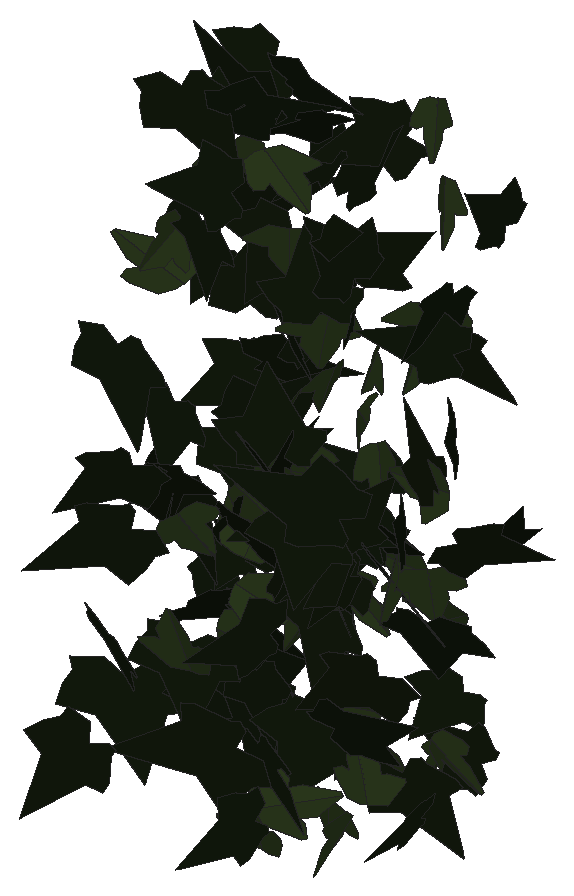
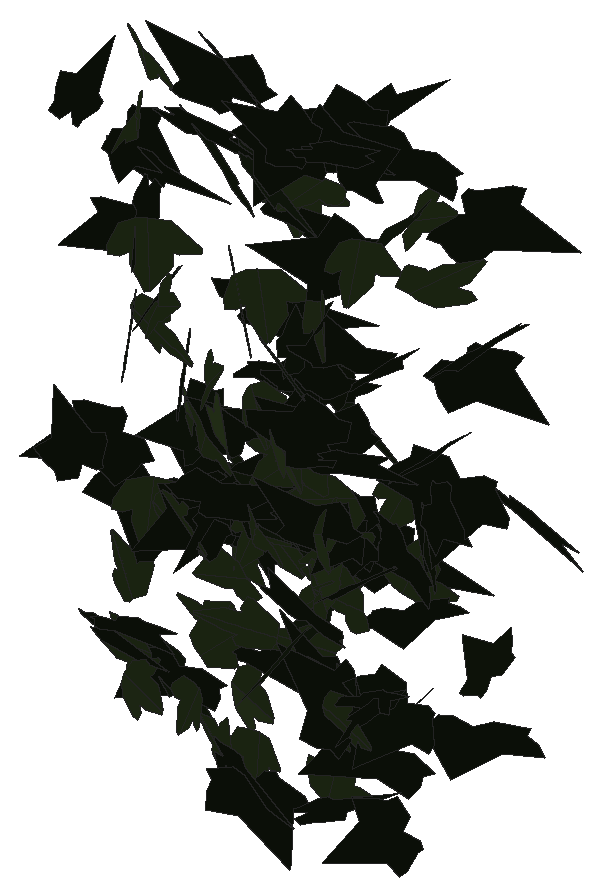
# SketchUp Ruby script. Lengths in inches.
U = 1.inch
M = Sketchup.active_model
def pt(a) = Geom::Point3d.new(a.map { |v| v * U })
def face(e, loops, mat)
  f = e.add_face(loops[0].map { |a| pt(a) })
  loops[1..].each { |l| e.add_face(l.map { |a| pt(a) }).erase! }
  f.material = f.back_material = mat if mat
  f
end
# faces: each face lists its corners as indices into pts; further lists are holes
def faces(e, pts, list, mat = nil) = list.each { |f| face(e, (f[0].is_a?(Array) ? f : [f]).map { |l| l.map { |i| pts[i] } }, mat) }
# xy, xz, yz: faces in a plane at the given z, y or x. An outline is a flat list of corners, or four numbers for a rectangle; further outlines are holes
def ring(l) = l.size == 4 ? [[l[0], l[1]], [l[2], l[1]], [l[2], l[3]], [l[0], l[3]]] : l.each_slice(2).to_a
def flat(e, list, mat, &to3) = list.each { |f| face(e, (f[0].is_a?(Array) ? f : [f]).map { |l| ring(l).map { |u, v| to3.(u, v) } }, mat) }
def xy(e, z, list, mat = nil) = flat(e, list, mat) { |x, y| [x, y, z] }
def xz(e, y, list, mat = nil) = flat(e, list, mat) { |x, z| [x, y, z] }
def yz(e, x, list, mat = nil) = flat(e, list, mat) { |y, z| [x, y, z] }
def lines(e, pts, list) = list.each { |a, b| e.add_line(pt(pts[a]), pt(pts[b])) }
# prism: a flat outline (further loops are holes) pulled along v
def prism(e, loops, v, mat = nil)
  f = face(e, loops, mat); d = Geom::Vector3d.new(v.map { |x| x * U })
  f.pushpull(f.normal.samedirection?(d) ? d.length : -d.length)
end
def box(e, o, s, mat = nil) = prism(e, [[o, [o[0] + s[0], o[1], o[2]], [o[0] + s[0], o[1] + s[1], o[2]], [o[0], o[1] + s[1], o[2]]]], [0, 0, s[2]], mat)
def at(x, y, z, deg = 0) = Geom::Transformation.translation(pt([x, y, z])) * Geom::Transformation.rotation(ORIGIN, Z_AXIS, deg.degrees)
def axes(o, x, y, z) = Geom::Transformation.new([*x, 0, *y, 0, *z, 0, *pt(o).to_a, 1])
def part(name) = M.definitions.add(name)
# library, detail: a bought-in or finely detailed component or shape, given as its bounding box
def library(name, o, s) = part(name).tap { |d| box(d.entities, o, s) }
def detail(e, o, s) = box(e.add_group.entities, o, s)
def put(e, d, t, mat = nil) = e.add_instance(d, t).tap { |i| i.material = mat if mat }
def group(e, t, mat = nil) = e.add_group.tap { |g| g.transformation = t; g.material = mat if mat }.entities
root = M.entities
M.materials.add("1026 AP 7946 SUNNY SIDE UP").color = [254, 231, 186]
M.materials.add("efeu1").color = [18, 25, 13]
M.materials.add("efeu2").color = [43, 57, 29]
c1 = part("ivyleaf_9")
p = [[1.54,2.16,1.25],[1.36,2.04,1.19],[-0.21,0.99,0.68],[-0.71,1.11,0.82],[-0.85,0.86,0.67],[-0.8,0.17,0.21],
  [-0.9,-0.01,0.1],[-0.67,-0.16,-0.02],[-0.08,-0.08,-0.05],[-0.03,-0.6,-0.4],[0.65,-0.88,-0.66],[0.83,-0.6,-0.49],
  [1.29,-0.42,-0.43],[1.8125,-0.07,-0.26],[1.21,0.44,0.15]]
faces(c1.entities,p,[[0,1,2,3,4,5,6,7,8,9,10,11,12,13,14]],"efeu1")
c2 = part("ivyleaf_10")
p = [[0,0.5,-0.03],[-0.0625,2.02,-0.43],[-0.19,2.01,-0.46],[-0.54,1.05,-0.29],[-0.52,0.625,-0.18],[-0.83,0.76,-0.28],
  [-1.16,0.64,-0.33],[-1.15,0.33,-0.24],[-0.77,-0.39,0.02],[-0.3,-0.51,0.16],[0.04,-0.48,0.23],[-0.02,2.01,-0.4375],
  [-0.06,2.01,-0.43],[0.04,-0.49,0.23],[0.67,-0.49,0.14],[1.38,0.36,-0.2],[1.375,0.51,-0.24],[0.81,0.65,-0.19],
  [0.62,0.59,-0.15],[0.6,1.09,-0.28],[0.5,1.23,-0.31]]
faces(c2.entities,p,[[0,1,2,3,4,5,6,7,8,9,10],[11,12,0,13,14,15,16,17,18,19,20]],"efeu2")
put(root,c1,axes([141.33,204.3125,274.67],[-0.08778,-0.02071,-0.48621],[-0.04144,-0.47425,0.02188],[-0.74149,0.02896,0.05633]),"1026 AP 7946 SUNNY SIDE UP")
put(root,c1,axes([140.3,204.62,270.57],[-0.70201,0.01951,-0.15809],[0.23469,-0.07018,-0.4566],[-0.0646,-0.46689,0.05923]),"1026 AP 7946 SUNNY SIDE UP")
put(root,c1,axes([142.83,205.35,269.84],[-0.60155,0.20655,-0.09318],[0.095,-0.08009,-0.44638],[-0.34235,-0.38515,0.03986]),"1026 AP 7946 SUNNY SIDE UP")
put(root,c1,axes([141.66,206.34,270.23],[-0.1412,-0.10196,-0.47524],[-0.44551,-0.3634,0.13761],[-0.59335,0.29712,0.00977]),"1026 AP 7946 SUNNY SIDE UP")
put(root,c1,axes([142.4375,206.1875,272.47],[-0.54529,0.329,0.00208],[-0.03997,-0.02658,-0.49115],[-0.51578,-0.34577,0.03587]),"1026 AP 7946 SUNNY SIDE UP")
put(root,c1,axes([139.4375,206.72,273.99],[0.00936,0.11052,-0.39414],[-0.09937,-0.37816,-0.11558],[-0.61921,0.06236,0.01259]),"1026 AP 7946 SUNNY SIDE UP")
put(root,c1,axes([142.97,207.22,270.625],[0.58209,0.0655,-0.17186],[0.22809,0.11671,0.37867],[0.16642,-0.38907,0.08211]),"1026 AP 7946 SUNNY SIDE UP")
put(root,c1,axes([141.375,207.39,269.68],[0.2811,-0.36238,0.03312],[-0.00053,-0.03828,-0.41613],[0.57235,0.17794,-0.01666]),"1026 AP 7946 SUNNY SIDE UP")
put(root,c1,axes([142.76,207.38,274.05],[-0.27783,0.07056,0.43166],[-0.65081,0.07215,-0.19208],[-0.14837,-0.44861,0.03424]),"1026 AP 7946 SUNNY SIDE UP")
put(root,c2,axes([139.95,207.39,270.67],[-0.56819,0.04904,-0.0988],[-0.14095,0.05096,0.37402],[0.0946,0.37045,-0.03612]),"1026 AP 7946 SUNNY SIDE UP")
put(root,c2,axes([141.7,207.24,268.91],[0.23552,-0.00672,-0.37454],[0.52266,0.16187,0.13896],[0.23169,-0.35831,0.06727]),"1026 AP 7946 SUNNY SIDE UP")
put(root,c1,axes([142.05,207.64,273.49],[-0.32105,-0.33925,-0.05283],[0.06514,0.03261,-0.40727],[0.5351,-0.20751,0.01788]),"1026 AP 7946 SUNNY SIDE UP")
put(root,c1,axes([138.36,207.82,275.13],[0.01346,-0.47992,0.01511],[0.01074,-0.01727,-0.49454],[0.75505,0.0088,0.00676]),"1026 AP 7946 SUNNY SIDE UP")
put(root,c1,axes([139.62,207.92,270.54],[-0.23506,-0.40184,-0.07874],[0.04593,0.06824,-0.44128],[0.64088,-0.15228,0.00275]),"1026 AP 7946 SUNNY SIDE UP")
put(root,c1,axes([138.04,207.99,270.125],[0.09553,-0.26086,0.27989],[0.13003,-0.26078,-0.27703],[0.57951,0.10151,0.01602]),"1026 AP 7946 SUNNY SIDE UP")
put(root,c1,axes([143.1,207.92,271.24],[0.09585,0.06198,-0.39943],[-0.34043,-0.32245,-0.08997],[-0.51571,0.22437,-0.01485]),"1026 AP 7946 SUNNY SIDE UP")
put(root,c1,axes([140.16,208.125,278.26],[-0.19778,-0.06121,0.4093],[-0.42491,-0.29581,-0.1367],[0.46869,-0.29401,0.04878]),"1026 AP 7946 SUNNY SIDE UP")
put(root,c2,axes([142.33,208.1,268.39],[0.1333,-0.29257,0.2564],[0.08138,-0.24556,-0.31489],[0.60018,0.09828,-0.01425]),"1026 AP 7946 SUNNY SIDE UP")
put(root,c2,axes([139.09,208.25,277.16],[0.09776,0.14683,-0.37943],[-0.14773,-0.3576,-0.16493],[-0.60695,0.11069,-0.02097]),"1026 AP 7946 SUNNY SIDE UP")
put(root,c2,axes([139.48,207.95,272.59],[-0.26698,-0.28775,-0.20995],[0.21357,0.15342,-0.34158],[0.51006,-0.21486,0.03313]),"1026 AP 7946 SUNNY SIDE UP")
put(root,c1,axes([142.77,207.79,277.94],[-0.13686,0.27393,0.38347],[-0.27002,0.33079,-0.29144],[-0.67255,-0.18855,0.03898]),"1026 AP 7946 SUNNY SIDE UP")
put(root,c1,axes([140.6875,208.06,274.11],[0.54317,-0.17404,-0.10493],[-0.16391,0.01655,-0.3971],[0.27051,0.35949,-0.02992]),"1026 AP 7946 SUNNY SIDE UP")
put(root,c1,axes([142.01,207.98,277.03],[-0.5582,-0.07882,0.12233],[0.16876,0.06367,0.37306],[-0.14835,0.36902,-0.03592]),"1026 AP 7946 SUNNY SIDE UP")
put(root,c1,axes([138.15,208.23,269.32],[-0.34763,-0.35399,-0.24935],[0.23608,0.18878,-0.42816],[0.62972,-0.26619,0.02286]),"1026 AP 7946 SUNNY SIDE UP")
put(root,c2,axes([142.84,208.04,269.21],[0.53812,-0.01345,0.14735],[-0.21966,0.0559,0.3499],[-0.05322,-0.36671,0.04573]),"1026 AP 7946 SUNNY SIDE UP")
put(root,c1,axes([138.57,208.05,273.03],[0.5327,0.28218,-0.10711],[-0.09377,-0.09292,-0.45354],[-0.46437,0.34247,-0.03129]),"1026 AP 7946 SUNNY SIDE UP")
put(root,c1,axes([142.54,208.16,277.88],[-0.15475,0.02402,0.40412],[0.59348,-0.10642,0.10368],[0.17146,0.39004,0.00586]),"1026 AP 7946 SUNNY SIDE UP")
put(root,c2,axes([140.62,208.26,267.5],[-0.53757,0.06449,-0.03595],[-0.04669,0.0323,0.35759],[0.10572,0.34217,-0.02489]),"1026 AP 7946 SUNNY SIDE UP")
put(root,c1,axes([141.7,208.55,271.54],[-0.15537,-0.37938,0.12184],[-0.03131,-0.11921,-0.40443],[0.62508,-0.10027,0.01003]),"1026 AP 7946 SUNNY SIDE UP")
put(root,c2,axes([143.15,208.12,272.3],[0.29387,-0.22552,0.26531],[-0.2243,0.21702,0.3022],[-0.49098,-0.23413,0.02074]),"1026 AP 7946 SUNNY SIDE UP")
put(root,c2,axes([138.74,208.52,276.25],[0.23187,0.26554,0.26408],[-0.25453,-0.19976,0.30976],[0.51973,-0.2163,0.03388]),"1026 AP 7946 SUNNY SIDE UP")
put(root,c1,axes([142.65,208.52,272.73],[0.472,-0.26867,0.0995],[0.07923,-0.09033,-0.41417],[0.44271,0.30261,-0.03197]),"1026 AP 7946 SUNNY SIDE UP")
put(root,c1,axes([141.5625,208.65,269.5],[-0.5956,-0.21258,-0.07549],[0.13602,-0.0078,-0.44472],[0.32568,-0.3855,0.04769]),"1026 AP 7946 SUNNY SIDE UP")
put(root,c1,axes([142.07,208.5625,272.25],[-0.45316,0.13622,-0.19567],[0.22888,-0.13286,-0.32515],[-0.28882,-0.31902,0.04933]),"1026 AP 7946 SUNNY SIDE UP")
put(root,c1,axes([143.46,208.49,268.74],[-0.37016,0.25797,-0.13574],[0.11149,-0.11524,-0.35963],[-0.44271,-0.24472,0.02293]),"1026 AP 7946 SUNNY SIDE UP")
put(root,c1,axes([142.04,208.76,272.22],[-0.21171,-0.21466,0.2554],[-0.18848,-0.21865,-0.2621],[0.48151,-0.17996,0.0097]),"1026 AP 7946 SUNNY SIDE UP")
put(root,c2,axes([141.34,208.68,271.5],[-0.10165,-0.32553,0.18508],[-0.02099,-0.18207,-0.34237],[0.58567,-0.06302,0.01985]),"1026 AP 7946 SUNNY SIDE UP")
put(root,c1,axes([139.12,208.82,277.07],[0.01819,-0.38176,0.18216],[0.00404,-0.17899,-0.39451],[0.66298,0.01156,-0.00259]),"1026 AP 7946 SUNNY SIDE UP")
put(root,c1,axes([141.09,208.3,272.05],[0.00352,0.18396,0.35024],[-0.02228,0.33874,-0.18734],[-0.60597,-0.01139,0.00892]),"1026 AP 7946 SUNNY SIDE UP")
put(root,c1,axes([142.92,208.8,273.07],[-0.03778,0.07812,0.3598],[-0.11961,-0.34271,0.07167],[0.54918,-0.06927,0.04036]),"1026 AP 7946 SUNNY SIDE UP")
put(root,c1,axes([138.8125,208.33,271.96],[-0.00393,0.02888,0.40579],[0.071,0.39118,-0.02698],[-0.6167,0.04485,-0.00569]),"1026 AP 7946 SUNNY SIDE UP")
put(root,c1,axes([138.5,208.92,273.77],[-0.09727,-0.37358,0.14709],[-0.02988,-0.14372,-0.39091],[0.62934,-0.06456,0.00417]),"1026 AP 7946 SUNNY SIDE UP")
put(root,c1,axes([140.78,208.54,273.97],[-0.57491,-0.0912,0.16107],[0.23203,0.0559,0.38813],[-0.16603,0.39391,-0.01531]),"1026 AP 7946 SUNNY SIDE UP")
put(root,c1,axes([138.37,208.82,273.06],[-0.2007,0.12443,-0.32054],[0.31131,-0.24156,-0.18418],[-0.42639,-0.23493,0.0164]),"1026 AP 7946 SUNNY SIDE UP")
put(root,c1,axes([143.86,208.6875,276.61],[-0.39161,0.12928,0.25636],[-0.38266,0.06376,-0.28551],[-0.21702,-0.34572,0.04083]),"1026 AP 7946 SUNNY SIDE UP")
put(root,c1,axes([139.125,209.02,269.19],[0.17762,-0.2802,-0.22578],[0.15576,-0.19434,0.30969],[-0.53563,-0.14943,0.01518]),"1026 AP 7946 SUNNY SIDE UP")
put(root,c2,axes([141.09,208.52,272.3125],[0.15454,0.01027,-0.38752],[-0.32787,0.32519,-0.04507],[0.49267,0.21319,0.09157]),"1026 AP 7946 SUNNY SIDE UP")
put(root,c1,axes([143.5625,208.66,274.3],[-0.15825,-0.27823,0.28306],[0.11036,0.26791,0.30579],[-0.60666,0.12132,-0.01821]),"1026 AP 7946 SUNNY SIDE UP")
put(root,c2,axes([141,208.76,273.41],[-0.58887,0.07318,-0.0741],[0.10129,-0.04621,-0.39196],[-0.12619,-0.37862,0.03119]),"1026 AP 7946 SUNNY SIDE UP")
put(root,c1,axes([139.68,208.85,272.16],[0.57429,-0.16064,0.1972],[0.24833,-0.11639,-0.40979],[0.30593,0.39603,-0.03754]),"1026 AP 7946 SUNNY SIDE UP")
put(root,c1,axes([140.79,208.48,273.54],[0.03377,0.10674,0.43817],[0.26161,0.39136,-0.1077],[-0.63697,0.16639,-0.021]),"1026 AP 7946 SUNNY SIDE UP")
put(root,c1,axes([138.72,209.01,272.29],[-0.2018,-0.05634,-0.41322],[0.63639,-0.02104,-0.13059],[-0.00481,-0.42031,0.05942]),"1026 AP 7946 SUNNY SIDE UP")
put(root,c1,axes([140.05,208.97,269.76],[-0.31353,-0.05901,-0.32266],[0.49225,0.03089,-0.21136],[0.09117,-0.36971,0.0316]),"1026 AP 7946 SUNNY SIDE UP")
put(root,c1,axes([143.61,209.05,277.3],[-0.11365,0.14194,-0.36763],[0.23252,-0.32572,-0.16586],[-0.55858,-0.16446,0.00575]),"1026 AP 7946 SUNNY SIDE UP")
put(root,c2,axes([143.55,208.74,274.22],[0.13498,-0.12002,-0.37317],[-0.44601,0.22726,-0.14577],[0.39986,0.29401,-0.03662]),"1026 AP 7946 SUNNY SIDE UP")
put(root,c2,axes([141.56,208.8125,268.13],[-0.47815,0.14381,0.06997],[-0.11414,0.00293,-0.34533],[-0.22191,-0.31139,0.02686]),"1026 AP 7946 SUNNY SIDE UP")
put(root,c1,axes([141.14,208.5625,271.84],[-0.33674,0.24858,-0.24937],[-0.2091,0.20572,0.33808],[0.50559,0.25064,-0.02627]),"1026 AP 7946 SUNNY SIDE UP")
put(root,c2,axes([140.73,208.89,277.375],[-0.4632,-0.21263,0.00481],[0.0193,-0.02701,-0.37323],[0.33392,-0.2934,0.02824]),"1026 AP 7946 SUNNY SIDE UP")
put(root,c1,axes([141.84,208.72,272.87],[-0.18998,-0.03852,0.35846],[0.49055,0.15567,0.13018],[-0.2505,0.33405,-0.01693]),"1026 AP 7946 SUNNY SIDE UP")
put(root,c2,axes([139.92,208.98,272.7],[-0.32259,0.0313,-0.32034],[0.45626,-0.11964,-0.21021],[-0.18326,-0.35295,0.04053]),"1026 AP 7946 SUNNY SIDE UP")
put(root,c2,axes([140.07,208.76,271.22],[0.13487,0.22376,0.26759],[0.16524,0.23633,-0.24531],[-0.51155,0.13533,-0.00869]),"1026 AP 7946 SUNNY SIDE UP")
put(root,c1,axes([142.8,208.99,269],[-0.16714,-0.17706,-0.3564],[0.39561,0.24065,-0.20572],[0.4639,-0.26902,0.04703]),"1026 AP 7946 SUNNY SIDE UP")
put(root,c2,axes([141.75,208.84,271.16],[-0.297,0.19682,-0.25507],[-0.23578,0.19967,0.28127],[0.43947,0.24014,-0.02148]),"1026 AP 7946 SUNNY SIDE UP")
put(root,c2,axes([142.02,209.23,269.71],[-0.14968,-0.09732,-0.31929],[-0.28128,-0.2532,0.13727],[-0.42539,0.20167,0.02158]),"1026 AP 7946 SUNNY SIDE UP")
put(root,c1,axes([139.97,209.15,269.71],[-0.045,0.07556,0.36657],[0.27315,-0.31027,0.08056],[0.50179,0.17567,-0.01098]),"1026 AP 7946 SUNNY SIDE UP")
put(root,c1,axes([143.26,208.97,271.72],[0.50042,0.20049,-0.19467],[-0.22327,-0.13006,-0.38697],[-0.37267,0.34714,-0.02956]),"1026 AP 7946 SUNNY SIDE UP")
put(root,c1,axes([140.41,209.27,277.18],[-0.58202,-0.14266,-0.10119],[0.16388,-0.00073,-0.40689],[0.21663,-0.38275,0.03594]),"1026 AP 7946 SUNNY SIDE UP")
put(root,c2,axes([139.87,208.97,271.88],[0.33375,0.22988,-0.18811],[0.14832,0.16165,0.32128],[0.43849,-0.22965,0.0345]),"1026 AP 7946 SUNNY SIDE UP")
put(root,c1,axes([141.14,209.27,271.82],[-0.125,-0.02486,-0.34638],[0.52959,-0.01765,-0.08083],[-0.01809,-0.34491,0.02707]),"1026 AP 7946 SUNNY SIDE UP")
put(root,c1,axes([139.66,208.91,272.37],[-0.0797,0.06272,-0.36329],[-0.22573,0.32313,0.08227],[0.51659,0.15087,-0.0201]),"1026 AP 7946 SUNNY SIDE UP")
put(root,c1,axes([138.45,209.25,278.89],[-0.22644,-0.17934,-0.39584],[0.50785,0.21491,-0.22739],[0.42978,-0.34844,0.06014]),"1026 AP 7946 SUNNY SIDE UP")
put(root,c1,axes([138.92,209.22,269.15],[-0.06761,-0.12362,-0.41265],[0.42863,0.29674,-0.12298],[0.49937,-0.27144,0.04968]),"1026 AP 7946 SUNNY SIDE UP")
put(root,c2,axes([141.07,209.3125,275.85],[-0.39123,-0.30557,0.02655],[0.00043,-0.03564,-0.40549],[0.48242,-0.24778,0.02189]),"1026 AP 7946 SUNNY SIDE UP")
put(root,c1,axes([140.52,209.53,272.4],[-0.45244,-0.14052,0.17362],[-0.21126,-0.10855,-0.32865],[0.27401,-0.31573,0.03329]),"1026 AP 7946 SUNNY SIDE UP")
put(root,c2,axes([143.17,209.44,269.37],[-0.16186,0.06557,-0.35466],[0.4073,-0.22802,-0.12573],[-0.37203,-0.27817,0.01666]),"1026 AP 7946 SUNNY SIDE UP")
put(root,c2,axes([139.2,209.45,269.92],[0.05677,-0.05771,-0.39558],[0.49181,-0.22366,0.06367],[-0.36096,-0.31381,0.02453]),"1026 AP 7946 SUNNY SIDE UP")
put(root,c2,axes([141.11,209.23,272.07],[-0.17931,-0.3021,-0.21568],[0.16301,0.182,-0.33038],[0.55288,-0.15164,0.02746]),"1026 AP 7946 SUNNY SIDE UP")
put(root,c2,axes([142.21,209.42,268.93],[-0.35925,0.23643,-0.04575],[0.02233,-0.04973,-0.33809],[-0.37799,-0.22764,0.02351]),"1026 AP 7946 SUNNY SIDE UP")
put(root,c2,axes([140.33,209.43,273.42],[-0.48016,-0.04613,-0.20747],[0.32235,-0.02692,-0.31446],[0.03694,-0.36466,0.04728]),"1026 AP 7946 SUNNY SIDE UP")
put(root,c1,axes([143.84,209.4,269.42],[-0.36193,-0.03513,-0.28423],[-0.43614,0.00628,0.23777],[-0.02778,0.3591,-0.02984]),"1026 AP 7946 SUNNY SIDE UP")
put(root,c1,axes([139.33,209.29,278.78],[0.20843,0.0684,0.39739],[0.59308,0.08626,-0.14893],[-0.16424,0.39828,-0.03348]),"1026 AP 7946 SUNNY SIDE UP")
put(root,c1,axes([140.41,209.5,275.06],[0.0833,-0.30932,0.24963],[-0.05374,0.24173,0.32466],[-0.61722,-0.06279,0.00542]),"1026 AP 7946 SUNNY SIDE UP")
put(root,c1,axes([139.73,209.34,273.7],[-0.16162,-0.02666,0.42593],[0.6201,0.12478,0.10998],[-0.20046,0.4075,-0.00319]),"1026 AP 7946 SUNNY SIDE UP")
put(root,c1,axes([143.02,209.49,276.17],[-0.03299,-0.0537,-0.37798],[0.39531,0.26765,-0.05365],[0.42794,-0.25138,0.02042]),"1026 AP 7946 SUNNY SIDE UP")
put(root,c1,axes([143.02,209.36,276.66],[0.06073,-0.0828,-0.38594],[-0.43261,0.25577,-0.08608],[0.41943,0.2758,-0.0329]),"1026 AP 7946 SUNNY SIDE UP")
put(root,c2,axes([142.77,209.58,272.06],[-0.40303,-0.28632,-0.05333],[0.08288,0.01996,-0.39489],[0.44948,-0.26041,0.02499]),"1026 AP 7946 SUNNY SIDE UP")
put(root,c2,axes([141.17,209.67,271.3125],[0.28251,0.02391,0.32278],[0.49347,-0.02833,-0.18342],[0.02006,0.35995,-0.03375]),"1026 AP 7946 SUNNY SIDE UP")
put(root,c2,axes([139.47,209.84,271.6],[-0.20455,-0.00325,0.37911],[0.46732,-0.23115,0.10477],[0.34132,0.31453,0.08375]),"1026 AP 7946 SUNNY SIDE UP")
put(root,c2,axes([139.85,209.58,278.01],[0.37085,0.19626,0.19185],[0.25842,0.09047,-0.314],[-0.33641,0.28584,-0.02971]),"1026 AP 7946 SUNNY SIDE UP")
put(root,c1,axes([141.65,209.72,272.17],[-0.10858,0.04689,0.37155],[-0.57022,0.01521,-0.07353],[-0.03755,-0.36663,0.04228]),"1026 AP 7946 SUNNY SIDE UP")
put(root,c2,axes([141.35,209.8,268.55],[-0.11968,0.03996,0.31799],[0.42899,-0.1439,0.08772],[0.23483,0.28324,0.00182]),"1026 AP 7946 SUNNY SIDE UP")
put(root,c1,axes([142.97,209.94,274.24],[-0.00228,-0.00371,0.38119],[-0.09507,-0.36507,-0.00615],[0.57406,-0.06048,0.0005]),"1026 AP 7946 SUNNY SIDE UP")
put(root,c1,axes([138.42,209.41,270.13],[0.30093,0.32516,0.17191],[0.14086,0.13873,-0.38783],[-0.55579,0.21122,-0.00521]),"1026 AP 7946 SUNNY SIDE UP")
put(root,c2,axes([142.83,209.91,269.15],[0.03884,-0.27974,0.22575],[0.04863,-0.21873,-0.29044],[0.55819,0.03852,0.0096]),"1026 AP 7946 SUNNY SIDE UP")
put(root,c1,axes([139.1,209.93,269.96],[0.45837,-0.1028,-0.36464],[0.56618,-0.0135,0.30998],[-0.1196,-0.45789,0.0699]),"1026 AP 7946 SUNNY SIDE UP")
put(root,c2,axes([141.5,209.92,273.5],[0.39484,-0.12918,0.26444],[0.32635,-0.15564,-0.28994],[0.31401,0.32419,-0.03119]),"1026 AP 7946 SUNNY SIDE UP")
put(root,c1,axes([143.05,209.96,270.06],[-0.45317,-0.14066,0.02072],[-0.00968,-0.03487,-0.32927],[0.22339,-0.28685,0.02776]),"1026 AP 7946 SUNNY SIDE UP")
put(root,c2,axes([142.65,209.84,276.34],[-0.44428,-0.27959,0.00217],[0.0279,-0.02317,-0.40855],[0.43878,-0.28162,0.02818]),"1026 AP 7946 SUNNY SIDE UP")
put(root,c1,axes([139.23,210.08,274.03],[-0.50142,-0.13679,0.16603],[-0.20284,-0.10691,-0.35534],[0.2645,-0.3413,0.04226]),"1026 AP 7946 SUNNY SIDE UP")
put(root,c2,axes([138.85,209.96,271.77],[0.10417,-0.04676,0.35708],[0.53239,-0.08092,-0.07833],[0.1395,0.34375,0.03229]),"1026 AP 7946 SUNNY SIDE UP")
put(root,c1,axes([141.27,209.66,276.1875],[0.01034,-0.03704,-0.42912],[-0.59909,0.17068,-0.02084],[0.27025,0.37979,-0.02979]),"1026 AP 7946 SUNNY SIDE UP")
put(root,c2,axes([139.3,210.14,272.83],[0.06473,-0.17256,0.35829],[0.26479,-0.30827,-0.17941],[0.55159,0.16823,0.04407]),"1026 AP 7946 SUNNY SIDE UP")
put(root,c1,axes([139.3,209.75,275.4375],[-0.48875,-0.03272,0.21255],[0.31944,0.04025,0.32181],[-0.07775,0.371,-0.01395]),"1026 AP 7946 SUNNY SIDE UP")
put(root,c2,axes([142.24,210.09,275.47],[0.0164,0.19324,-0.31893],[-0.0405,-0.30965,-0.20111],[-0.57388,0.02738,0.00508]),"1026 AP 7946 SUNNY SIDE UP")
put(root,c1,axes([143.36,209.61,272.8125],[0.02724,0.12919,-0.38519],[0.09077,0.37017,0.13642],[0.61647,-0.06021,-0.00306]),"1026 AP 7946 SUNNY SIDE UP")
put(root,c1,axes([138.37,210.16,275.76],[-0.16201,-0.28313,0.17038],[-0.07932,-0.15931,-0.31126],[0.51074,-0.11455,0.0057]),"1026 AP 7946 SUNNY SIDE UP")
put(root,c1,axes([139.32,209.76,278.62],[0.09288,-0.03131,0.44287],[-0.39757,0.34911,0.064],[-0.54923,-0.25801,0.02856]),"1026 AP 7946 SUNNY SIDE UP")
put(root,c1,axes([141.39,209.73,272.25],[0.0919,-0.10387,-0.33306],[-0.18921,0.29979,-0.12011],[0.49836,0.13298,0.01582]),"1026 AP 7946 SUNNY SIDE UP")
put(root,c2,axes([142.36,209.77,271.98],[0.10621,-0.10209,-0.35668],[-0.3996,0.23586,-0.12155],[0.40183,0.26154,-0.0266]),"1026 AP 7946 SUNNY SIDE UP")
put(root,c1,axes([143.74,210.13,278.1],[0.06518,0.08789,0.38461],[-0.36837,-0.29089,0.09578],[0.47654,-0.23688,0.02143]),"1026 AP 7946 SUNNY SIDE UP")
put(root,c1,axes([141.57,209.88,272.21],[0.567,-0.04227,0.04287],[0.05871,-0.03931,-0.37256],[0.07281,0.36088,-0.0334]),"1026 AP 7946 SUNNY SIDE UP")
put(root,c2,axes([142.72,210.08,278.3],[-0.03197,0.31728,-0.22841],[0.0087,-0.22357,-0.32875],[-0.6102,-0.01981,0.00728]),"1026 AP 7946 SUNNY SIDE UP")
put(root,c2,axes([140.43,210.14,272.54],[0.39203,-0.14241,0.27826],[0.3295,-0.17526,-0.2946],[0.35077,0.32379,-0.03425]),"1026 AP 7946 SUNNY SIDE UP")
put(root,c1,axes([140.64,210.04,278.27],[-0.49212,0.21352,-0.14607],[0.14779,-0.11461,-0.38891],[-0.37609,-0.32444,0.0383]),"1026 AP 7946 SUNNY SIDE UP")
put(root,c2,axes([140.57,210.02,274.52],[-0.03831,-0.33915,0.00563],[0.00876,-0.00781,-0.35028],[0.53334,-0.02423,0.00616]),"1026 AP 7946 SUNNY SIDE UP")
put(root,c1,axes([139.85,209.83,271.18],[-0.43958,0.21948,0.14994],[0.20003,-0.07124,0.36511],[0.36135,0.30644,-0.01971]),"1026 AP 7946 SUNNY SIDE UP")
put(root,c1,axes([139.2,209.73,276.96],[0.09226,0.06136,0.4271],[0.58078,0.18949,-0.08171],[-0.31023,0.37299,-0.02595]),"1026 AP 7946 SUNNY SIDE UP")
put(root,c1,axes([140.38,209.8,275.11],[-0.33933,0.06708,-0.26999],[-0.37628,0.11005,0.23233],[0.19962,0.32147,-0.02101]),"1026 AP 7946 SUNNY SIDE UP")
put(root,c2,axes([140.07,210.12,274.1],[0.14427,-0.37987,0.06496],[0.00842,-0.06578,-0.40284],[0.60599,0.09135,-0.00987]),"1026 AP 7946 SUNNY SIDE UP")
put(root,c1,axes([140.1,209.82,278.7],[0.34911,0.27214,0.03173],[0.04345,0.01519,-0.36153],[-0.42818,0.22342,-0.01082]),"1026 AP 7946 SUNNY SIDE UP")
put(root,c2,axes([140.97,210.29,273.87],[-0.01649,-0.1371,-0.31467],[0.14454,-0.29424,0.13143],[-0.50506,-0.07973,0.04789]),"1026 AP 7946 SUNNY SIDE UP")
put(root,c2,axes([140.54,209.97,270.8],[-0.0594,0.00813,0.33766],[0.44707,0.16502,0.03051],[-0.25658,0.28565,-0.02501]),"1026 AP 7946 SUNNY SIDE UP")
put(root,c1,axes([141.01,209.97,277.82],[-0.17604,0.362,0.18019],[0.077,-0.16578,0.38938],[0.62605,0.12218,0.00278]),"1026 AP 7946 SUNNY SIDE UP")
put(root,c2,axes([142.35,210.22,279.48],[0.41144,-0.1448,0.18416],[0.21434,-0.12202,-0.30669],[0.29263,0.29296,-0.03428]),"1026 AP 7946 SUNNY SIDE UP")
put(root,c1,axes([139.34,210.05,272.79],[-0.09093,0.00938,0.33209],[0.48998,-0.0825,0.05959],[0.13026,0.31688,0.00767]),"1026 AP 7946 SUNNY SIDE UP")
put(root,c1,axes([141.11,209.99,268.55],[-0.19423,-0.01832,-0.38022],[-0.58088,0.00673,0.12711],[0.0009,0.38904,-0.01782]),"1026 AP 7946 SUNNY SIDE UP")
put(root,c1,axes([138.33,210.08,270.49],[0.13758,-0.24728,-0.19735],[-0.07429,0.18471,-0.26877],[0.48484,0.09847,0.01482]),"1026 AP 7946 SUNNY SIDE UP")
put(root,c2,axes([139.21,209.96,269.95],[0.02655,-0.04661,-0.36385],[-0.38355,0.25582,-0.04533],[0.4077,0.24371,-0.01895]),"1026 AP 7946 SUNNY SIDE UP")
put(root,c1,axes([139.35,210.32,268.49],[-0.16589,-0.29219,-0.1605],[-0.09714,-0.1415,0.31907],[-0.51028,0.12192,-0.00856]),"1026 AP 7946 SUNNY SIDE UP")
put(root,c1,axes([138.16,209.86,268.38],[0.28273,0.20497,0.25791],[0.29797,0.1638,-0.27871],[-0.41063,0.25999,-0.02467]),"1026 AP 7946 SUNNY SIDE UP")
put(root,c2,axes([139.5625,209.95,276.36],[-0.26497,0.16412,0.31207],[-0.36963,0.19034,-0.24058],[-0.39428,-0.28873,0.01582]),"1026 AP 7946 SUNNY SIDE UP")
put(root,c1,axes([139.34,210.08,274.27],[0.22723,0.00101,0.33986],[0.51439,-0.0469,-0.14776],[0.06692,0.35709,-0.01824]),"1026 AP 7946 SUNNY SIDE UP")
put(root,c1,axes([139.93,210.14,270.75],[0.30713,-0.28372,-0.18868],[-0.15683,0.15173,-0.35395],[0.50589,0.21929,0.00482]),"1026 AP 7946 SUNNY SIDE UP")
put(root,c1,axes([138.51,210.33,272.44],[0.01192,-0.37806,-0.0218],[0.05704,0.01966,-0.38761],[0.59248,0.00572,0.03776]),"1026 AP 7946 SUNNY SIDE UP")
put(root,c1,axes([140.52,210.15,268.44],[0.29312,0.15714,-0.30202],[-0.32116,-0.21247,-0.2516],[-0.41438,0.27583,-0.01865]),"1026 AP 7946 SUNNY SIDE UP")
put(root,c1,axes([143.56,210.2,272.57],[0.29226,0.24062,0.16138],[-0.17941,-0.10758,0.31179],[0.41302,-0.217,0.02124]),"1026 AP 7946 SUNNY SIDE UP")
put(root,c2,axes([141.14,210.41,274.76],[-0.00478,0.08451,-0.32469],[0.00188,-0.31567,-0.08892],[-0.51382,-0.00194,0.00269]),"1026 AP 7946 SUNNY SIDE UP")
put(root,c2,axes([142.57,210.3,270.97],[-0.35919,0.09198,0.26799],[0.3634,-0.11945,0.2524],[0.23557,0.32452,0.01925]),"1026 AP 7946 SUNNY SIDE UP")
put(root,c1,axes([139.64,210.27,279.01],[0.2261,-0.09167,0.30407],[0.35307,-0.19355,-0.17544],[0.33509,0.26579,-0.02032]),"1026 AP 7946 SUNNY SIDE UP")
put(root,c1,axes([139.16,210.42,279.15],[-0.48409,-0.16076,0.12654],[-0.13885,-0.09629,-0.35575],[0.2872,-0.31753,0.04131]),"1026 AP 7946 SUNNY SIDE UP")
put(root,c2,axes([138.63,210.16,277.5625],[-0.28139,-0.31074,-0.09597],[0.1106,0.06464,-0.36793],[0.49716,-0.19026,0.02753]),"1026 AP 7946 SUNNY SIDE UP")
put(root,c1,axes([138.42,210.37,270.67],[-0.26432,-0.211,0.02861],[-0.00757,-0.03313,-0.27757],[0.3348,-0.16733,0.01631]),"1026 AP 7946 SUNNY SIDE UP")
put(root,c1,axes([141.3,210.26,272.74],[-0.06337,0.0835,0.36974],[-0.57751,0.01378,-0.04577],[-0.03676,-0.36042,0.08168]),"1026 AP 7946 SUNNY SIDE UP")
put(root,c1,axes([141.66,210.34,278.75],[-0.62507,0.03897,0.10532],[-0.16668,-0.04505,-0.40805],[-0.04131,-0.40793,0.05269]),"1026 AP 7946 SUNNY SIDE UP")
